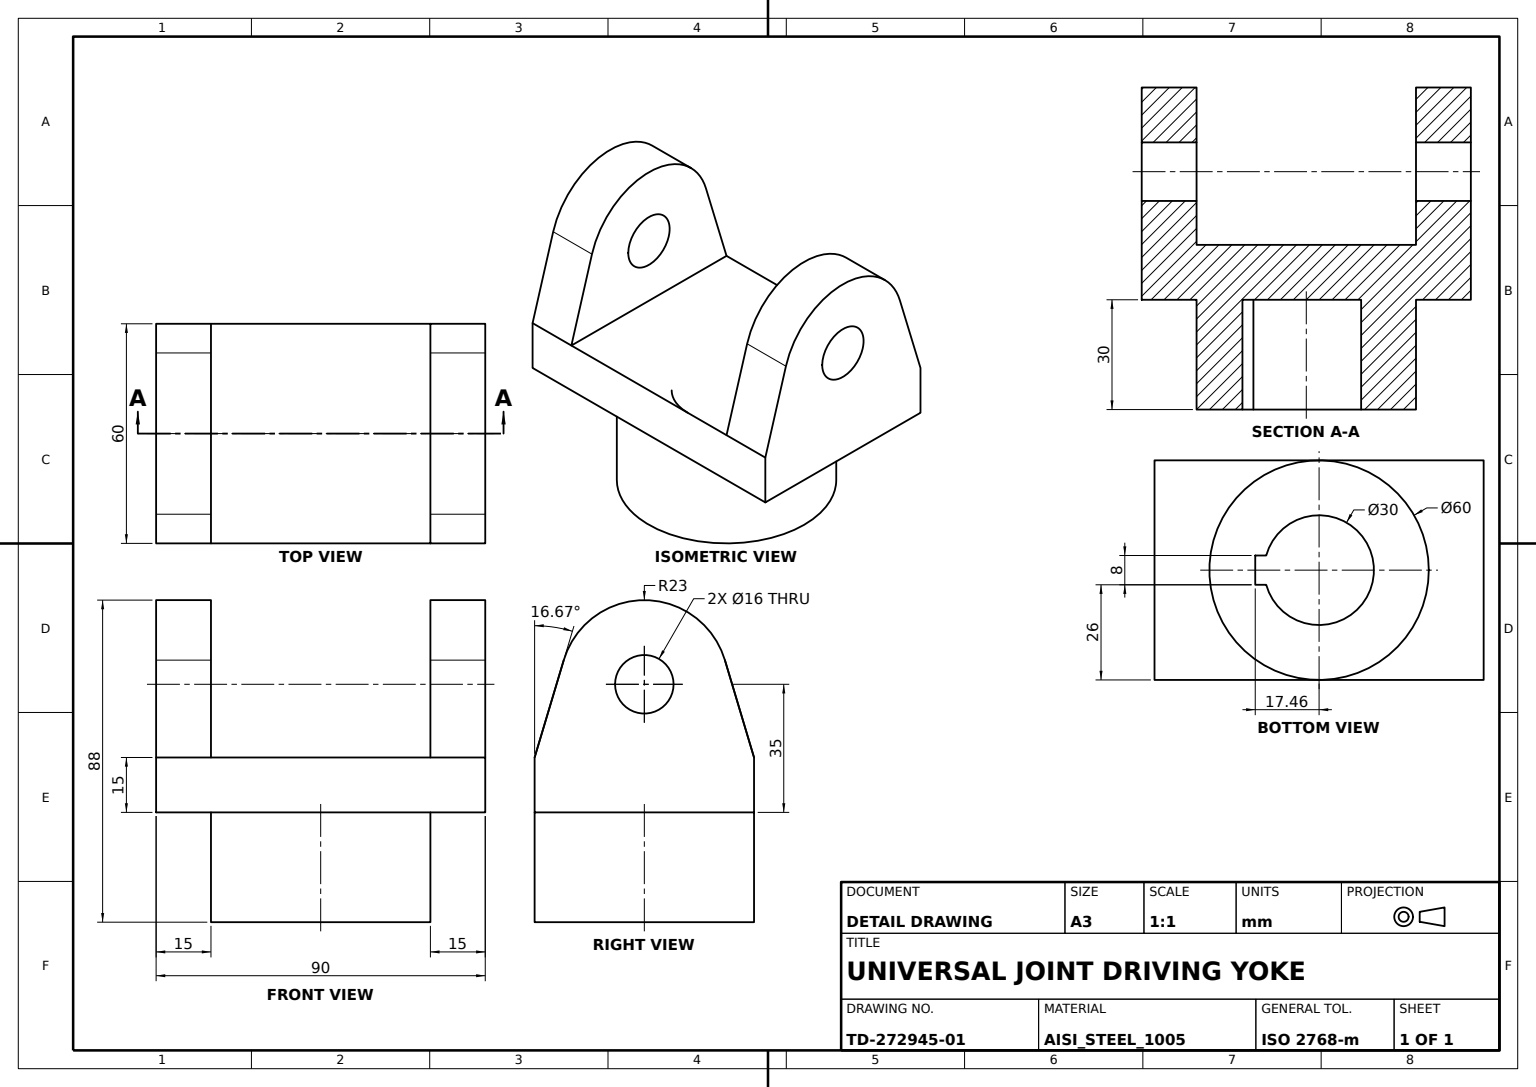
ISO-10303-21;
HEADER;
FILE_DESCRIPTION((''),'2;1');
FILE_NAME('','',(''),(''),'','','');
FILE_SCHEMA(('AUTOMOTIVE_DESIGN'));
ENDSEC;
DATA;
#1=APPLICATION_CONTEXT('');
#2=PRODUCT_CONTEXT('',#1,'mechanical');
#3=PRODUCT('','','',(#2));
#4=PRODUCT_DEFINITION_FORMATION('','',#3);
#5=PRODUCT_DEFINITION_CONTEXT('',#1,'design');
#6=PRODUCT_DEFINITION('','',#4,#5);
#7=PRODUCT_DEFINITION_SHAPE('','',#6);
#8=(LENGTH_UNIT()NAMED_UNIT(*)SI_UNIT(.MILLI.,.METRE.));
#9=(NAMED_UNIT(*)PLANE_ANGLE_UNIT()SI_UNIT($,.RADIAN.));
#10=(NAMED_UNIT(*)SI_UNIT($,.STERADIAN.)SOLID_ANGLE_UNIT());
#11=UNCERTAINTY_MEASURE_WITH_UNIT(LENGTH_MEASURE(0.005),#8,'distance_accuracy_value','');
#12=(GEOMETRIC_REPRESENTATION_CONTEXT(3)GLOBAL_UNCERTAINTY_ASSIGNED_CONTEXT((#11))GLOBAL_UNIT_ASSIGNED_CONTEXT((#8,#9,#10))REPRESENTATION_CONTEXT('',''));
#13=CARTESIAN_POINT('',(30.,30.,15.));
#14=VERTEX_POINT('',#13);
#15=CARTESIAN_POINT('',(-30.,30.,15.));
#16=VERTEX_POINT('',#15);
#17=CARTESIAN_POINT('',(45.,30.,15.));
#18=DIRECTION('',(-1.,0.,0.));
#19=VECTOR('',#18,1000.);
#20=LINE('',#17,#19);
#21=EDGE_CURVE('',#14,#16,#20,.T.);
#22=ORIENTED_EDGE('',*,*,#21,.F.);
#23=VERTEX_POINT('',#17);
#24=EDGE_CURVE('',#23,#14,#20,.T.);
#25=ORIENTED_EDGE('',*,*,#24,.F.);
#26=CARTESIAN_POINT('',(45.,30.,0.));
#27=VERTEX_POINT('',#26);
#28=DIRECTION('',(0.,0.,-1.));
#29=VECTOR('',#28,1000.);
#30=LINE('',#17,#29);
#31=EDGE_CURVE('',#23,#27,#30,.T.);
#32=ORIENTED_EDGE('',*,*,#31,.T.);
#33=CARTESIAN_POINT('',(0.,30.,0.));
#34=VERTEX_POINT('',#33);
#35=LINE('',#26,#19);
#36=EDGE_CURVE('',#27,#34,#35,.T.);
#37=ORIENTED_EDGE('',*,*,#36,.T.);
#38=CARTESIAN_POINT('',(-45.,30.,0.));
#39=VERTEX_POINT('',#38);
#40=EDGE_CURVE('',#34,#39,#35,.T.);
#41=ORIENTED_EDGE('',*,*,#40,.T.);
#42=CARTESIAN_POINT('',(-45.,30.,15.));
#43=VERTEX_POINT('',#42);
#44=LINE('',#42,#29);
#45=EDGE_CURVE('',#43,#39,#44,.T.);
#46=ORIENTED_EDGE('',*,*,#45,.F.);
#47=LINE('',#15,#19);
#48=EDGE_CURVE('',#16,#43,#47,.T.);
#49=ORIENTED_EDGE('',*,*,#48,.F.);
#50=EDGE_LOOP('',(#22,#25,#32,#37,#41,#46,#49));
#51=FACE_BOUND('',#50,.T.);
#52=DIRECTION('',(0.,-1.,0.));
#53=AXIS2_PLACEMENT_3D('',#17,#52,#28);
#54=PLANE('',#53);
#55=ADVANCED_FACE('',(#51),#54,.F.);
#56=CARTESIAN_POINT('',(-45.,-30.,15.));
#57=VERTEX_POINT('',#56);
#58=CARTESIAN_POINT('',(-30.,-30.,15.));
#59=VERTEX_POINT('',#58);
#60=DIRECTION('',(1.,0.,0.));
#61=VECTOR('',#60,1000.);
#62=LINE('',#56,#61);
#63=EDGE_CURVE('',#57,#59,#62,.T.);
#64=ORIENTED_EDGE('',*,*,#63,.F.);
#65=CARTESIAN_POINT('',(-45.,-30.,0.));
#66=VERTEX_POINT('',#65);
#67=LINE('',#56,#29);
#68=EDGE_CURVE('',#57,#66,#67,.T.);
#69=ORIENTED_EDGE('',*,*,#68,.T.);
#70=CARTESIAN_POINT('',(0.,-30.,0.));
#71=VERTEX_POINT('',#70);
#72=LINE('',#65,#61);
#73=EDGE_CURVE('',#66,#71,#72,.T.);
#74=ORIENTED_EDGE('',*,*,#73,.T.);
#75=CARTESIAN_POINT('',(45.,-30.,0.));
#76=VERTEX_POINT('',#75);
#77=EDGE_CURVE('',#71,#76,#72,.T.);
#78=ORIENTED_EDGE('',*,*,#77,.T.);
#79=CARTESIAN_POINT('',(45.,-30.,15.));
#80=VERTEX_POINT('',#79);
#81=LINE('',#79,#29);
#82=EDGE_CURVE('',#80,#76,#81,.T.);
#83=ORIENTED_EDGE('',*,*,#82,.F.);
#84=CARTESIAN_POINT('',(30.,-30.,15.));
#85=VERTEX_POINT('',#84);
#86=LINE('',#84,#61);
#87=EDGE_CURVE('',#85,#80,#86,.T.);
#88=ORIENTED_EDGE('',*,*,#87,.F.);
#89=EDGE_CURVE('',#59,#85,#62,.T.);
#90=ORIENTED_EDGE('',*,*,#89,.F.);
#91=EDGE_LOOP('',(#64,#69,#74,#78,#83,#88,#90));
#92=FACE_BOUND('',#91,.T.);
#93=DIRECTION('',(0.,1.,0.));
#94=DIRECTION('',(0.,0.,1.));
#95=AXIS2_PLACEMENT_3D('',#56,#93,#94);
#96=PLANE('',#95);
#97=ADVANCED_FACE('',(#92),#96,.F.);
#98=ORIENTED_EDGE('',*,*,#89,.T.);
#99=VECTOR('',#52,1000.);
#100=LINE('',#13,#99);
#101=EDGE_CURVE('',#14,#85,#100,.T.);
#102=ORIENTED_EDGE('',*,*,#101,.F.);
#103=ORIENTED_EDGE('',*,*,#21,.T.);
#104=LINE('',#15,#99);
#105=EDGE_CURVE('',#16,#59,#104,.T.);
#106=ORIENTED_EDGE('',*,*,#105,.T.);
#107=EDGE_LOOP('',(#98,#102,#103,#106));
#108=FACE_BOUND('',#107,.T.);
#109=CARTESIAN_POINT('',(0.,0.,15.));
#110=AXIS2_PLACEMENT_3D('',#109,#94,#60);
#111=PLANE('',#110);
#112=ADVANCED_FACE('',(#108),#111,.T.);
#113=CARTESIAN_POINT('',(-17.456832,-4.,0.));
#114=VERTEX_POINT('',#113);
#115=CARTESIAN_POINT('',(-17.456832,4.,0.));
#116=VERTEX_POINT('',#115);
#117=VECTOR('',#93,1000.);
#118=LINE('',#113,#117);
#119=EDGE_CURVE('',#114,#116,#118,.T.);
#120=ORIENTED_EDGE('',*,*,#119,.T.);
#121=CARTESIAN_POINT('',(-14.456832,4.,0.));
#122=VERTEX_POINT('',#121);
#123=LINE('',#115,#61);
#124=EDGE_CURVE('',#116,#122,#123,.T.);
#125=ORIENTED_EDGE('',*,*,#124,.T.);
#126=CARTESIAN_POINT('',(-14.456832,-4.,0.));
#127=VERTEX_POINT('',#126);
#128=CARTESIAN_POINT('',(0.,0.,0.));
#129=AXIS2_PLACEMENT_3D('',#128,#28,#60);
#130=CIRCLE('',#129,15.);
#131=EDGE_CURVE('',#122,#127,#130,.T.);
#132=ORIENTED_EDGE('',*,*,#131,.T.);
#133=LINE('',#126,#19);
#134=EDGE_CURVE('',#127,#114,#133,.T.);
#135=ORIENTED_EDGE('',*,*,#134,.T.);
#136=EDGE_LOOP('',(#120,#125,#132,#135));
#137=FACE_BOUND('',#136,.T.);
#138=AXIS2_PLACEMENT_3D('',#128,#94,#60);
#139=PLANE('',#138);
#140=ADVANCED_FACE('',(#137),#139,.F.);
#141=CARTESIAN_POINT('',(-14.456832,4.,-30.));
#142=VERTEX_POINT('',#141);
#143=CARTESIAN_POINT('',(-14.456832,-4.,-30.));
#144=VERTEX_POINT('',#143);
#145=CARTESIAN_POINT('',(0.,0.,-30.));
#146=AXIS2_PLACEMENT_3D('',#145,#28,#60);
#147=CIRCLE('',#146,15.);
#148=EDGE_CURVE('',#142,#144,#147,.T.);
#149=ORIENTED_EDGE('',*,*,#148,.T.);
#150=VECTOR('',#94,1000.);
#151=LINE('',#143,#150);
#152=EDGE_CURVE('',#144,#127,#151,.T.);
#153=ORIENTED_EDGE('',*,*,#152,.T.);
#154=ORIENTED_EDGE('',*,*,#131,.F.);
#155=LINE('',#141,#150);
#156=EDGE_CURVE('',#142,#122,#155,.T.);
#157=ORIENTED_EDGE('',*,*,#156,.F.);
#158=EDGE_LOOP('',(#149,#153,#154,#157));
#159=FACE_BOUND('',#158,.T.);
#160=AXIS2_PLACEMENT_3D('',#145,#94,#60);
#161=CYLINDRICAL_SURFACE('',#160,15.);
#162=ADVANCED_FACE('',(#159),#161,.F.);
#163=CARTESIAN_POINT('',(-30.,-8.,35.));
#164=VERTEX_POINT('',#163);
#165=CARTESIAN_POINT('',(-30.,0.,35.));
#166=AXIS2_PLACEMENT_3D('',#165,#18,#52);
#167=CIRCLE('',#166,8.);
#168=EDGE_CURVE('',#164,#164,#167,.T.);
#169=ORIENTED_EDGE('',*,*,#168,.F.);
#170=EDGE_LOOP('',(#169));
#171=FACE_BOUND('',#170,.T.);
#172=CARTESIAN_POINT('',(-45.,-8.,35.));
#173=VERTEX_POINT('',#172);
#174=CARTESIAN_POINT('',(-45.,0.,35.));
#175=AXIS2_PLACEMENT_3D('',#174,#18,#52);
#176=CIRCLE('',#175,8.);
#177=EDGE_CURVE('',#173,#173,#176,.T.);
#178=ORIENTED_EDGE('',*,*,#177,.T.);
#179=EDGE_LOOP('',(#178));
#180=FACE_BOUND('',#179,.T.);
#181=AXIS2_PLACEMENT_3D('',#165,#18,#94);
#182=CYLINDRICAL_SURFACE('',#181,8.);
#183=ADVANCED_FACE('',(#171,#180),#182,.F.);
#184=CARTESIAN_POINT('',(-17.456832,-4.,-30.));
#185=VERTEX_POINT('',#184);
#186=LINE('',#184,#150);
#187=EDGE_CURVE('',#185,#114,#186,.T.);
#188=ORIENTED_EDGE('',*,*,#187,.T.);
#189=ORIENTED_EDGE('',*,*,#134,.F.);
#190=ORIENTED_EDGE('',*,*,#152,.F.);
#191=LINE('',#143,#19);
#192=EDGE_CURVE('',#144,#185,#191,.T.);
#193=ORIENTED_EDGE('',*,*,#192,.T.);
#194=EDGE_LOOP('',(#188,#189,#190,#193));
#195=FACE_BOUND('',#194,.T.);
#196=AXIS2_PLACEMENT_3D('',#143,#93,#18);
#197=PLANE('',#196);
#198=ADVANCED_FACE('',(#195),#197,.T.);
#199=CARTESIAN_POINT('',(30.,-8.,35.));
#200=VERTEX_POINT('',#199);
#201=CARTESIAN_POINT('',(30.,0.,35.));
#202=AXIS2_PLACEMENT_3D('',#201,#18,#52);
#203=CIRCLE('',#202,8.);
#204=EDGE_CURVE('',#200,#200,#203,.T.);
#205=ORIENTED_EDGE('',*,*,#204,.F.);
#206=EDGE_LOOP('',(#205));
#207=FACE_BOUND('',#206,.T.);
#208=ORIENTED_EDGE('',*,*,#101,.T.);
#209=CARTESIAN_POINT('',(30.,-22.032898,41.599348));
#210=VERTEX_POINT('',#209);
#211=DIRECTION('',(0.,0.286928156,0.957952104));
#212=VECTOR('',#211,1000.);
#213=LINE('',#84,#212);
#214=EDGE_CURVE('',#85,#210,#213,.T.);
#215=ORIENTED_EDGE('',*,*,#214,.T.);
#216=CARTESIAN_POINT('',(30.,22.032898,41.599348));
#217=VERTEX_POINT('',#216);
#218=CIRCLE('',#202,23.);
#219=EDGE_CURVE('',#210,#217,#218,.T.);
#220=ORIENTED_EDGE('',*,*,#219,.T.);
#221=DIRECTION('',(0.,0.286928156,-0.957952104));
#222=VECTOR('',#221,1000.);
#223=LINE('',#216,#222);
#224=EDGE_CURVE('',#217,#14,#223,.T.);
#225=ORIENTED_EDGE('',*,*,#224,.T.);
#226=EDGE_LOOP('',(#208,#215,#220,#225));
#227=FACE_BOUND('',#226,.T.);
#228=AXIS2_PLACEMENT_3D('',#201,#18,#94);
#229=PLANE('',#228);
#230=ADVANCED_FACE('',(#207,#227),#229,.T.);
#231=CARTESIAN_POINT('',(-45.,-22.032898,41.599348));
#232=VERTEX_POINT('',#231);
#233=CARTESIAN_POINT('',(-45.,22.032898,41.599348));
#234=VERTEX_POINT('',#233);
#235=CIRCLE('',#175,23.);
#236=EDGE_CURVE('',#232,#234,#235,.T.);
#237=ORIENTED_EDGE('',*,*,#236,.F.);
#238=CARTESIAN_POINT('',(-30.,-22.032898,41.599348));
#239=VERTEX_POINT('',#238);
#240=LINE('',#238,#19);
#241=EDGE_CURVE('',#239,#232,#240,.T.);
#242=ORIENTED_EDGE('',*,*,#241,.F.);
#243=CARTESIAN_POINT('',(-30.,22.032898,41.599348));
#244=VERTEX_POINT('',#243);
#245=CIRCLE('',#166,23.);
#246=EDGE_CURVE('',#239,#244,#245,.T.);
#247=ORIENTED_EDGE('',*,*,#246,.T.);
#248=LINE('',#243,#19);
#249=EDGE_CURVE('',#244,#234,#248,.T.);
#250=ORIENTED_EDGE('',*,*,#249,.T.);
#251=EDGE_LOOP('',(#237,#242,#247,#250));
#252=FACE_BOUND('',#251,.T.);
#253=CYLINDRICAL_SURFACE('',#181,23.);
#254=ADVANCED_FACE('',(#252),#253,.T.);
#255=ORIENTED_EDGE('',*,*,#87,.T.);
#256=CARTESIAN_POINT('',(45.,-22.032898,41.599348));
#257=VERTEX_POINT('',#256);
#258=LINE('',#79,#212);
#259=EDGE_CURVE('',#80,#257,#258,.T.);
#260=ORIENTED_EDGE('',*,*,#259,.T.);
#261=LINE('',#209,#61);
#262=EDGE_CURVE('',#210,#257,#261,.T.);
#263=ORIENTED_EDGE('',*,*,#262,.F.);
#264=ORIENTED_EDGE('',*,*,#214,.F.);
#265=EDGE_LOOP('',(#255,#260,#263,#264));
#266=FACE_BOUND('',#265,.T.);
#267=DIRECTION('',(0.,0.957952104,-0.286928156));
#268=AXIS2_PLACEMENT_3D('',#84,#267,#211);
#269=PLANE('',#268);
#270=ADVANCED_FACE('',(#266),#269,.F.);
#271=ORIENTED_EDGE('',*,*,#63,.T.);
#272=LINE('',#58,#212);
#273=EDGE_CURVE('',#59,#239,#272,.T.);
#274=ORIENTED_EDGE('',*,*,#273,.T.);
#275=ORIENTED_EDGE('',*,*,#241,.T.);
#276=LINE('',#56,#212);
#277=EDGE_CURVE('',#57,#232,#276,.T.);
#278=ORIENTED_EDGE('',*,*,#277,.F.);
#279=EDGE_LOOP('',(#271,#274,#275,#278));
#280=FACE_BOUND('',#279,.T.);
#281=DIRECTION('',(0.,-0.957952104,0.286928156));
#282=DIRECTION('',(0.,-0.286928156,-0.957952104));
#283=AXIS2_PLACEMENT_3D('',#58,#281,#282);
#284=PLANE('',#283);
#285=ADVANCED_FACE('',(#280),#284,.T.);
#286=ORIENTED_EDGE('',*,*,#249,.F.);
#287=LINE('',#243,#222);
#288=EDGE_CURVE('',#244,#16,#287,.T.);
#289=ORIENTED_EDGE('',*,*,#288,.T.);
#290=ORIENTED_EDGE('',*,*,#48,.T.);
#291=LINE('',#233,#222);
#292=EDGE_CURVE('',#234,#43,#291,.T.);
#293=ORIENTED_EDGE('',*,*,#292,.F.);
#294=EDGE_LOOP('',(#286,#289,#290,#293));
#295=FACE_BOUND('',#294,.T.);
#296=DIRECTION('',(0.,0.957952104,0.286928156));
#297=DIRECTION('',(0.,-0.286928156,0.957952104));
#298=AXIS2_PLACEMENT_3D('',#243,#296,#297);
#299=PLANE('',#298);
#300=ADVANCED_FACE('',(#295),#299,.T.);
#301=ORIENTED_EDGE('',*,*,#204,.T.);
#302=EDGE_LOOP('',(#301));
#303=FACE_BOUND('',#302,.T.);
#304=CARTESIAN_POINT('',(45.,-8.,35.));
#305=VERTEX_POINT('',#304);
#306=CARTESIAN_POINT('',(45.,0.,35.));
#307=AXIS2_PLACEMENT_3D('',#306,#18,#52);
#308=CIRCLE('',#307,8.);
#309=EDGE_CURVE('',#305,#305,#308,.T.);
#310=ORIENTED_EDGE('',*,*,#309,.F.);
#311=EDGE_LOOP('',(#310));
#312=FACE_BOUND('',#311,.T.);
#313=AXIS2_PLACEMENT_3D('',#201,#60,#28);
#314=CYLINDRICAL_SURFACE('',#313,8.);
#315=ADVANCED_FACE('',(#303,#312),#314,.F.);
#316=ORIENTED_EDGE('',*,*,#187,.F.);
#317=CARTESIAN_POINT('',(-17.456832,4.,-30.));
#318=VERTEX_POINT('',#317);
#319=LINE('',#184,#117);
#320=EDGE_CURVE('',#185,#318,#319,.T.);
#321=ORIENTED_EDGE('',*,*,#320,.T.);
#322=LINE('',#317,#150);
#323=EDGE_CURVE('',#318,#116,#322,.T.);
#324=ORIENTED_EDGE('',*,*,#323,.T.);
#325=ORIENTED_EDGE('',*,*,#119,.F.);
#326=EDGE_LOOP('',(#316,#321,#324,#325));
#327=FACE_BOUND('',#326,.T.);
#328=AXIS2_PLACEMENT_3D('',#184,#60,#93);
#329=PLANE('',#328);
#330=ADVANCED_FACE('',(#327),#329,.T.);
#331=ORIENTED_EDGE('',*,*,#177,.F.);
#332=EDGE_LOOP('',(#331));
#333=FACE_BOUND('',#332,.T.);
#334=ORIENTED_EDGE('',*,*,#68,.F.);
#335=ORIENTED_EDGE('',*,*,#277,.T.);
#336=ORIENTED_EDGE('',*,*,#236,.T.);
#337=ORIENTED_EDGE('',*,*,#292,.T.);
#338=ORIENTED_EDGE('',*,*,#45,.T.);
#339=LINE('',#38,#99);
#340=EDGE_CURVE('',#39,#66,#339,.T.);
#341=ORIENTED_EDGE('',*,*,#340,.T.);
#342=EDGE_LOOP('',(#334,#335,#336,#337,#338,#341));
#343=FACE_BOUND('',#342,.T.);
#344=AXIS2_PLACEMENT_3D('',#42,#60,#93);
#345=PLANE('',#344);
#346=ADVANCED_FACE('',(#333,#343),#345,.F.);
#347=ORIENTED_EDGE('',*,*,#168,.T.);
#348=EDGE_LOOP('',(#347));
#349=FACE_BOUND('',#348,.T.);
#350=ORIENTED_EDGE('',*,*,#273,.F.);
#351=ORIENTED_EDGE('',*,*,#105,.F.);
#352=ORIENTED_EDGE('',*,*,#288,.F.);
#353=ORIENTED_EDGE('',*,*,#246,.F.);
#354=EDGE_LOOP('',(#350,#351,#352,#353));
#355=FACE_BOUND('',#354,.T.);
#356=PLANE('',#181);
#357=ADVANCED_FACE('',(#349,#355),#356,.F.);
#358=CIRCLE('',#138,30.);
#359=EDGE_CURVE('',#34,#71,#358,.T.);
#360=ORIENTED_EDGE('',*,*,#359,.T.);
#361=ORIENTED_EDGE('',*,*,#73,.F.);
#362=ORIENTED_EDGE('',*,*,#340,.F.);
#363=ORIENTED_EDGE('',*,*,#40,.F.);
#364=EDGE_LOOP('',(#360,#361,#362,#363));
#365=FACE_BOUND('',#364,.T.);
#366=ADVANCED_FACE('',(#365),#139,.F.);
#367=CARTESIAN_POINT('',(45.,22.032898,41.599348));
#368=VERTEX_POINT('',#367);
#369=LINE('',#367,#222);
#370=EDGE_CURVE('',#368,#23,#369,.T.);
#371=ORIENTED_EDGE('',*,*,#370,.T.);
#372=ORIENTED_EDGE('',*,*,#24,.T.);
#373=ORIENTED_EDGE('',*,*,#224,.F.);
#374=LINE('',#216,#61);
#375=EDGE_CURVE('',#217,#368,#374,.T.);
#376=ORIENTED_EDGE('',*,*,#375,.T.);
#377=EDGE_LOOP('',(#371,#372,#373,#376));
#378=FACE_BOUND('',#377,.T.);
#379=DIRECTION('',(0.,-0.957952104,-0.286928156));
#380=AXIS2_PLACEMENT_3D('',#216,#379,#221);
#381=PLANE('',#380);
#382=ADVANCED_FACE('',(#378),#381,.F.);
#383=EDGE_CURVE('',#71,#34,#358,.T.);
#384=ORIENTED_EDGE('',*,*,#383,.F.);
#385=ORIENTED_EDGE('',*,*,#359,.F.);
#386=EDGE_LOOP('',(#384,#385));
#387=FACE_BOUND('',#386,.T.);
#388=CARTESIAN_POINT('',(30.,0.,-30.));
#389=VERTEX_POINT('',#388);
#390=CIRCLE('',#160,30.);
#391=EDGE_CURVE('',#389,#389,#390,.T.);
#392=ORIENTED_EDGE('',*,*,#391,.T.);
#393=EDGE_LOOP('',(#392));
#394=FACE_BOUND('',#393,.T.);
#395=CYLINDRICAL_SURFACE('',#160,30.);
#396=ADVANCED_FACE('',(#387,#394),#395,.T.);
#397=ORIENTED_EDGE('',*,*,#77,.F.);
#398=ORIENTED_EDGE('',*,*,#383,.T.);
#399=ORIENTED_EDGE('',*,*,#36,.F.);
#400=LINE('',#75,#117);
#401=EDGE_CURVE('',#76,#27,#400,.T.);
#402=ORIENTED_EDGE('',*,*,#401,.F.);
#403=EDGE_LOOP('',(#397,#398,#399,#402));
#404=FACE_BOUND('',#403,.T.);
#405=ADVANCED_FACE('',(#404),#139,.F.);
#406=ORIENTED_EDGE('',*,*,#391,.F.);
#407=EDGE_LOOP('',(#406));
#408=FACE_BOUND('',#407,.T.);
#409=LINE('',#317,#61);
#410=EDGE_CURVE('',#318,#142,#409,.T.);
#411=ORIENTED_EDGE('',*,*,#410,.F.);
#412=ORIENTED_EDGE('',*,*,#320,.F.);
#413=ORIENTED_EDGE('',*,*,#192,.F.);
#414=ORIENTED_EDGE('',*,*,#148,.F.);
#415=EDGE_LOOP('',(#411,#412,#413,#414));
#416=FACE_BOUND('',#415,.T.);
#417=PLANE('',#160);
#418=ADVANCED_FACE('',(#408,#416),#417,.F.);
#419=CIRCLE('',#307,23.);
#420=EDGE_CURVE('',#257,#368,#419,.T.);
#421=ORIENTED_EDGE('',*,*,#420,.T.);
#422=ORIENTED_EDGE('',*,*,#375,.F.);
#423=ORIENTED_EDGE('',*,*,#219,.F.);
#424=ORIENTED_EDGE('',*,*,#262,.T.);
#425=EDGE_LOOP('',(#421,#422,#423,#424));
#426=FACE_BOUND('',#425,.T.);
#427=CYLINDRICAL_SURFACE('',#313,23.);
#428=ADVANCED_FACE('',(#426),#427,.T.);
#429=ORIENTED_EDGE('',*,*,#124,.F.);
#430=ORIENTED_EDGE('',*,*,#323,.F.);
#431=ORIENTED_EDGE('',*,*,#410,.T.);
#432=ORIENTED_EDGE('',*,*,#156,.T.);
#433=EDGE_LOOP('',(#429,#430,#431,#432));
#434=FACE_BOUND('',#433,.T.);
#435=AXIS2_PLACEMENT_3D('',#317,#52,#28);
#436=PLANE('',#435);
#437=ADVANCED_FACE('',(#434),#436,.T.);
#438=ORIENTED_EDGE('',*,*,#309,.T.);
#439=EDGE_LOOP('',(#438));
#440=FACE_BOUND('',#439,.T.);
#441=ORIENTED_EDGE('',*,*,#370,.F.);
#442=ORIENTED_EDGE('',*,*,#420,.F.);
#443=ORIENTED_EDGE('',*,*,#259,.F.);
#444=ORIENTED_EDGE('',*,*,#82,.T.);
#445=ORIENTED_EDGE('',*,*,#401,.T.);
#446=ORIENTED_EDGE('',*,*,#31,.F.);
#447=EDGE_LOOP('',(#441,#442,#443,#444,#445,#446));
#448=FACE_BOUND('',#447,.T.);
#449=AXIS2_PLACEMENT_3D('',#79,#18,#52);
#450=PLANE('',#449);
#451=ADVANCED_FACE('',(#440,#448),#450,.F.);
#452=CLOSED_SHELL('',(#55,#97,#112,#140,#162,#183,#198,#230,#254,#270,#285,#300,#315,#330,#346,#357,#366,#382,#396,#405,#418,#428,#437,#451));
#453=MANIFOLD_SOLID_BREP('',#452);
#454=ADVANCED_BREP_SHAPE_REPRESENTATION('',(#453),#12);
#455=SHAPE_DEFINITION_REPRESENTATION(#7,#454);
ENDSEC;
END-ISO-10303-21;
